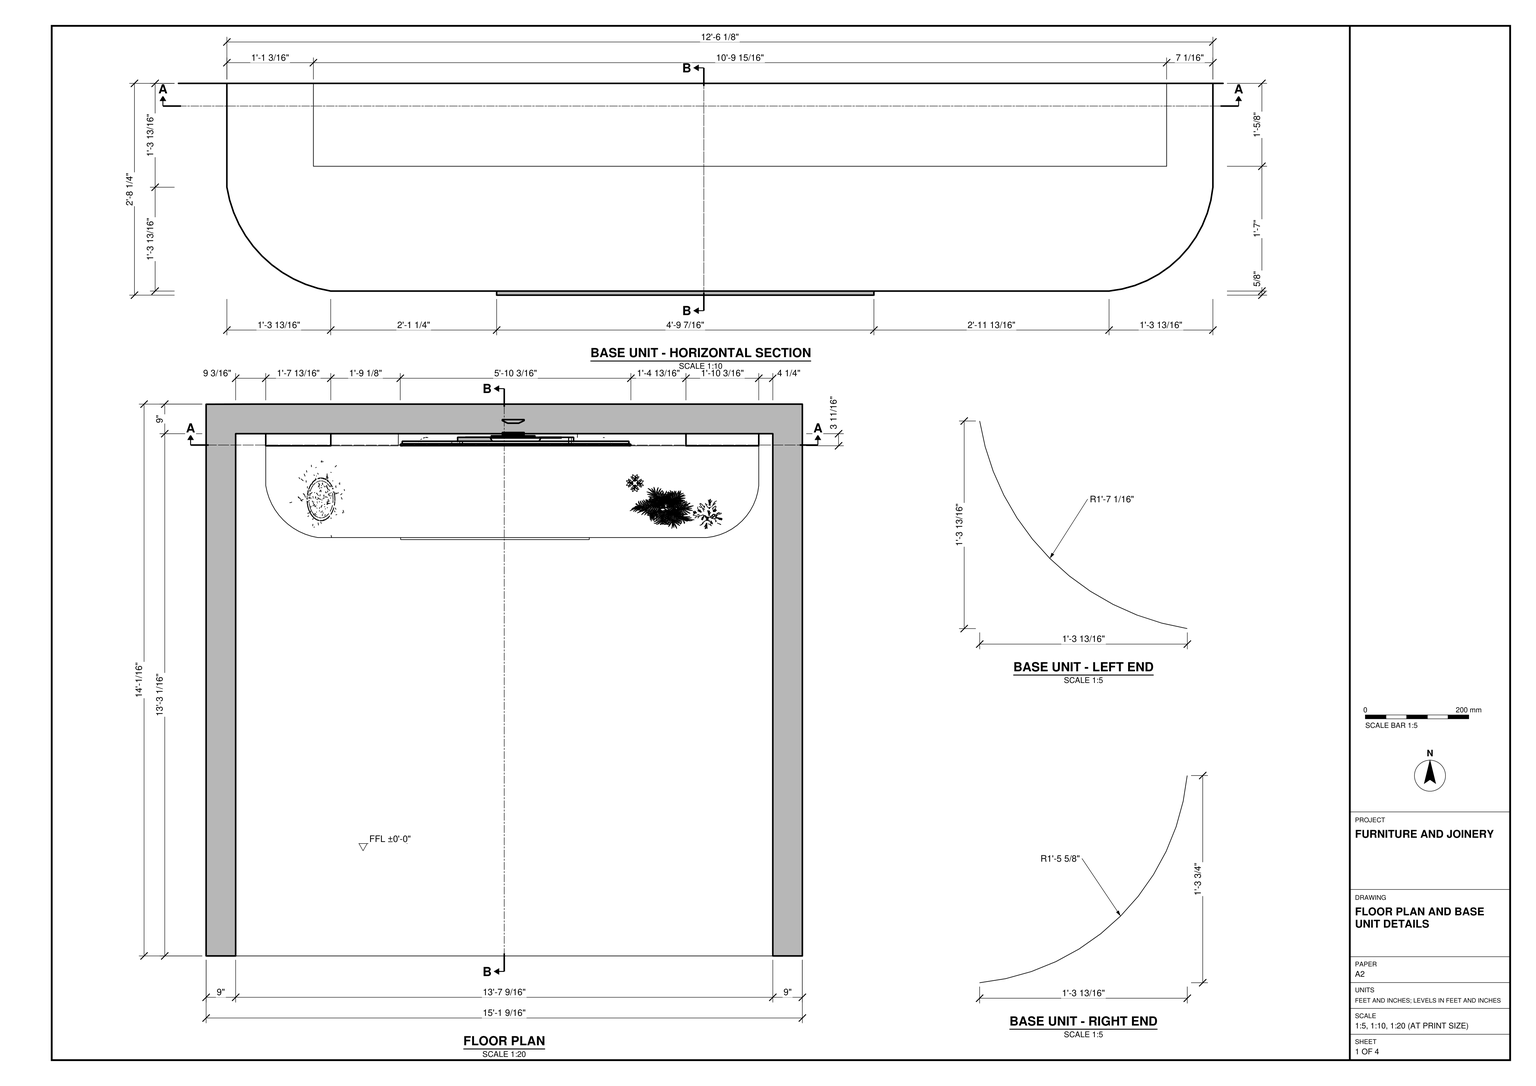
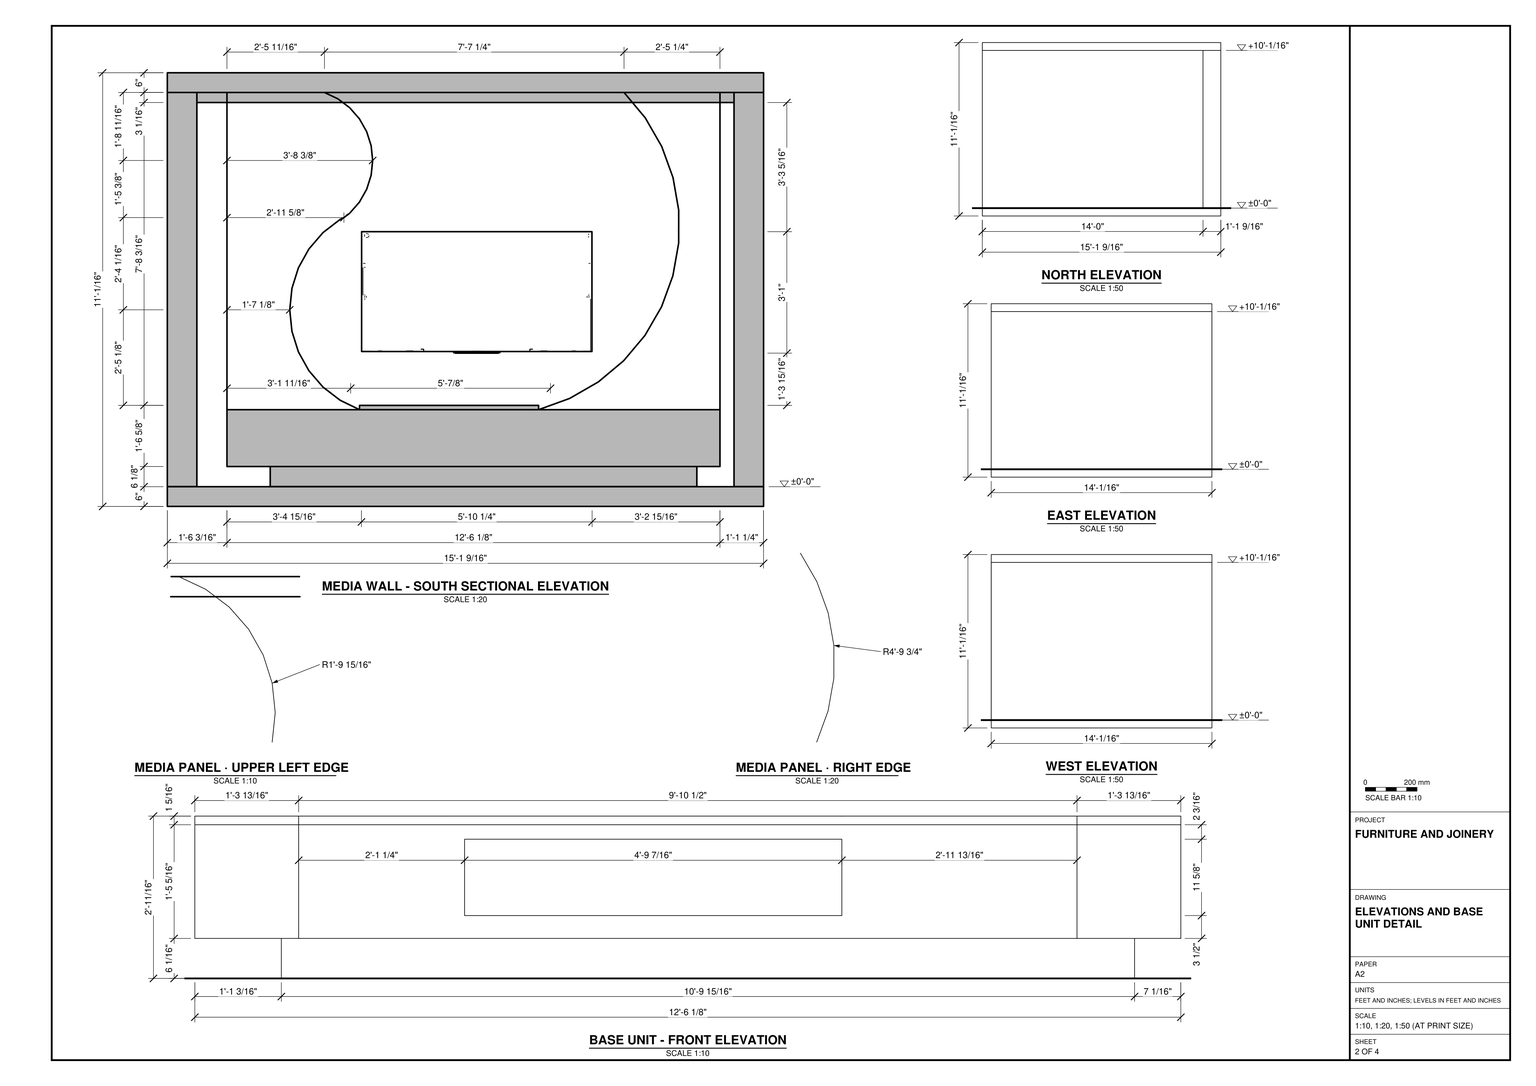
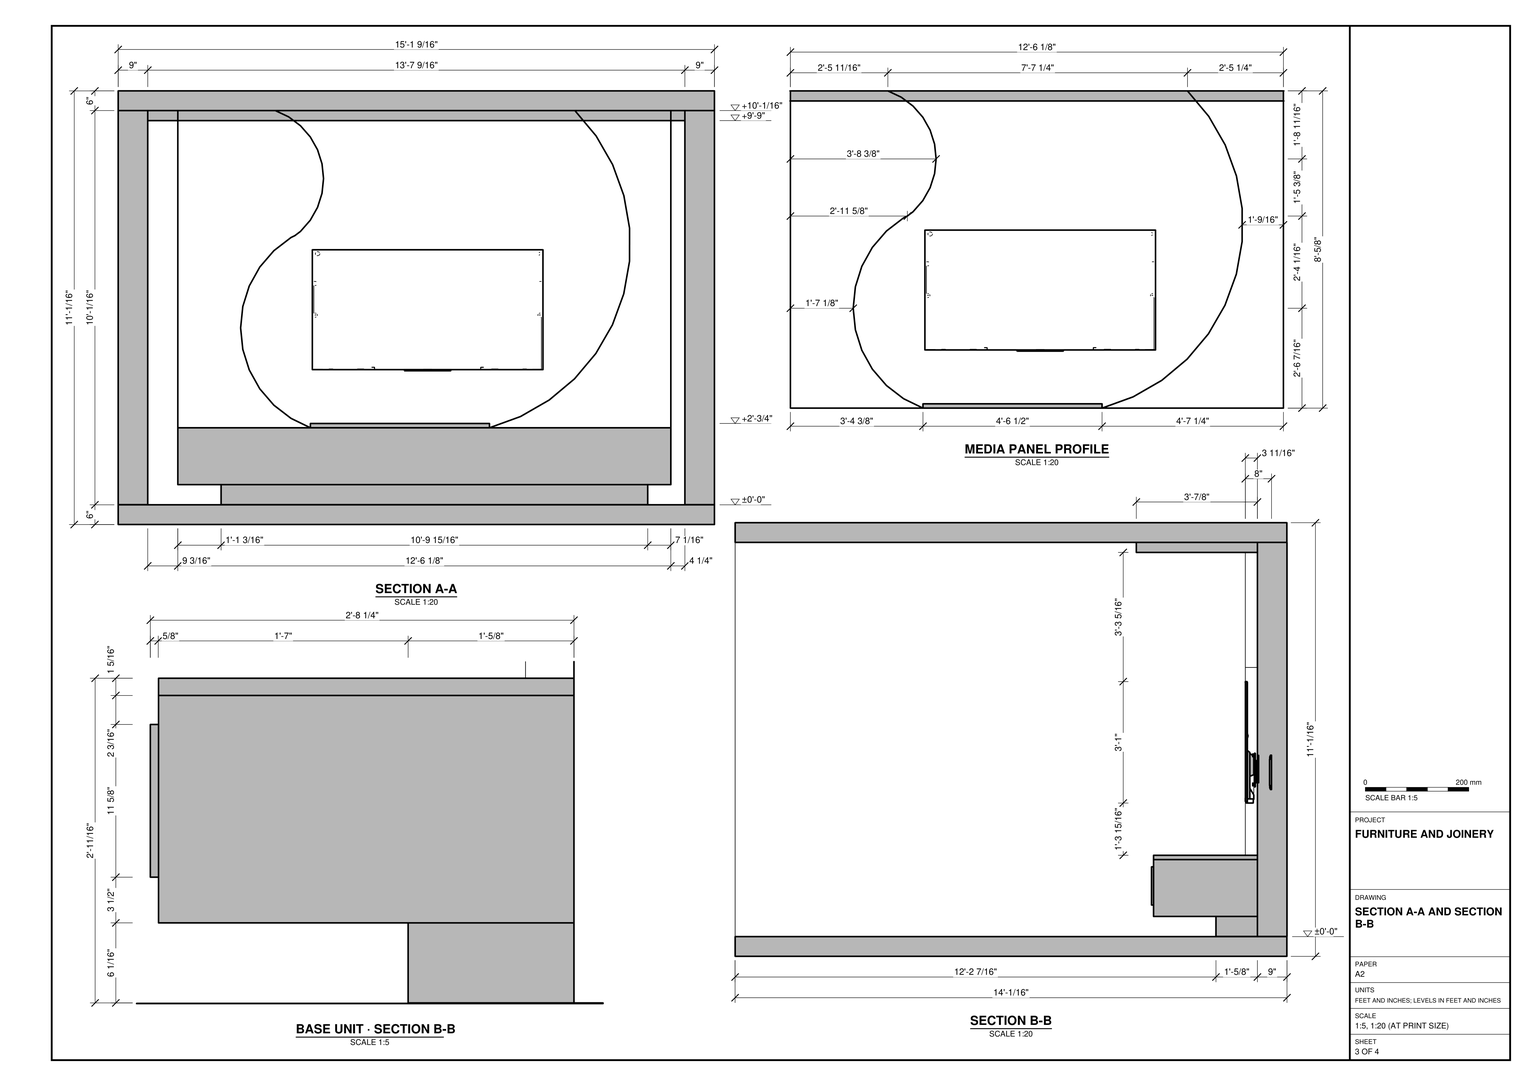
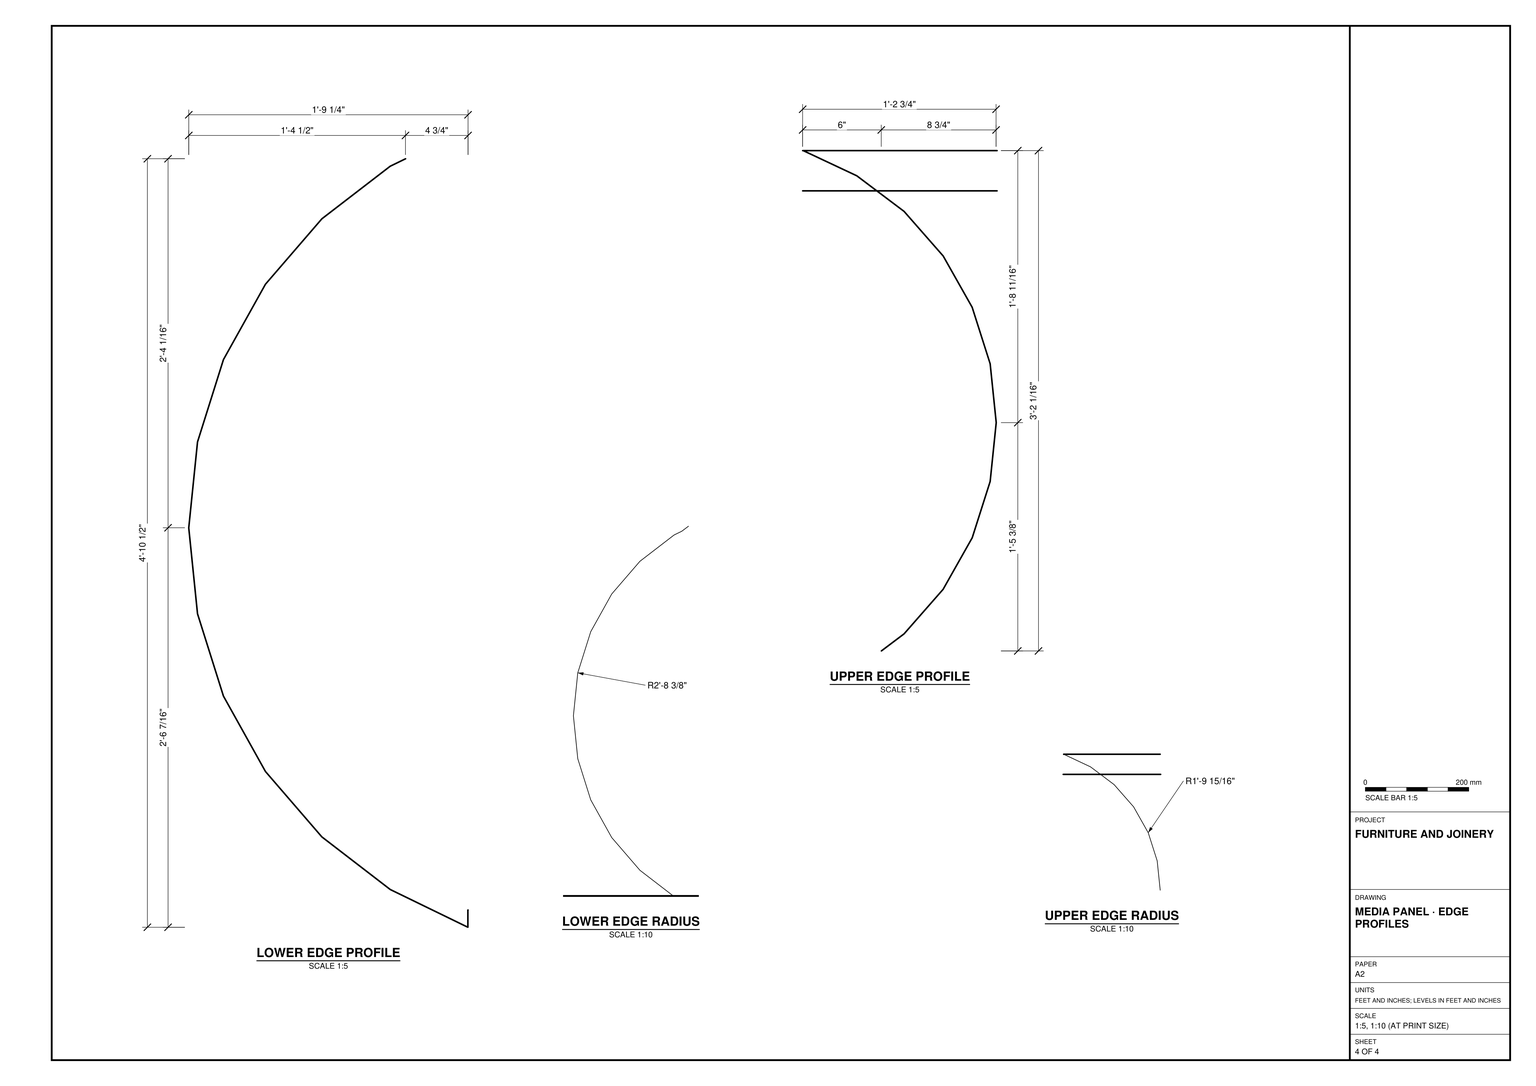
Build the media wall and its surrounding room shell in SketchUp using task_files/diagram_01.pdf. Work in feet and inches. The overall model is 15'-1 9/16" wide, 14'-1/16" deep and 11'-1/16" high, with the finished floor at ±0'-0". Form the floor slab, back wall, side walls and overhead slab, leaving the front open as shown. Use the 9" wall thickness and the slab thicknesses shown in section.

Place the base unit against the back wall, preserving the unequal clearances at its ends. Use the horizontal section and end details to shape the rounded front corners. Include the top, the projecting rectangular front panel and the recessed plinth. Above the unit, follow the media panel profile: the left edge reverses curvature, while the right edge sweeps out in a broad bow. Position the screen in front of the panel and model the shallow overhead projection shown in section. Decor and loose items, including the objects on the base unit, may be any suitable library components.

Keep the shell elements and each furniture or joinery piece in separate groups or components, and use components for repeated parts. Save one SketchUp model as output_files/media_wall_and_its_curved_base_unit.skp.

# SketchUp Ruby script. Lengths in inches.
U = 1.inch
M = Sketchup.active_model
def pt(a) = Geom::Point3d.new(a.map { |v| v * U })
def face(e, loops, mat)
  f = e.add_face(loops[0].map { |a| pt(a) })
  loops[1..].each { |l| e.add_face(l.map { |a| pt(a) }).erase! }
  f.material = f.back_material = mat if mat
  f
end
# faces: each face lists its corners as indices into pts; further lists are holes
def faces(e, pts, list, mat = nil) = list.each { |f| face(e, (f[0].is_a?(Array) ? f : [f]).map { |l| l.map { |i| pts[i] } }, mat) }
# xy, xz, yz: faces in a plane at the given z, y or x. An outline is a flat list of corners, or four numbers for a rectangle; further outlines are holes
def ring(l) = l.size == 4 ? [[l[0], l[1]], [l[2], l[1]], [l[2], l[3]], [l[0], l[3]]] : l.each_slice(2).to_a
def flat(e, list, mat, &to3) = list.each { |f| face(e, (f[0].is_a?(Array) ? f : [f]).map { |l| ring(l).map { |u, v| to3.(u, v) } }, mat) }
def xy(e, z, list, mat = nil) = flat(e, list, mat) { |x, y| [x, y, z] }
def xz(e, y, list, mat = nil) = flat(e, list, mat) { |x, z| [x, y, z] }
def yz(e, x, list, mat = nil) = flat(e, list, mat) { |y, z| [x, y, z] }
def lines(e, pts, list) = list.each { |a, b| e.add_line(pt(pts[a]), pt(pts[b])) }
# prism: a flat outline (further loops are holes) pulled along v
def prism(e, loops, v, mat = nil)
  f = face(e, loops, mat); d = Geom::Vector3d.new(v.map { |x| x * U })
  f.pushpull(f.normal.samedirection?(d) ? d.length : -d.length)
end
def box(e, o, s, mat = nil) = prism(e, [[o, [o[0] + s[0], o[1], o[2]], [o[0] + s[0], o[1] + s[1], o[2]], [o[0], o[1] + s[1], o[2]]]], [0, 0, s[2]], mat)
def at(x, y, z, deg = 0) = Geom::Transformation.translation(pt([x, y, z])) * Geom::Transformation.rotation(ORIGIN, Z_AXIS, deg.degrees)
def axes(o, x, y, z) = Geom::Transformation.new([*x, 0, *y, 0, *z, 0, *pt(o).to_a, 1])
def part(name) = M.definitions.add(name)
# library, detail: a bought-in or finely detailed component or shape, given as its bounding box
def library(name, o, s) = part(name).tap { |d| box(d.entities, o, s) }
def detail(e, o, s) = box(e.add_group.entities, o, s)
def put(e, d, t, mat = nil) = e.add_instance(d, t).tap { |i| i.material = mat if mat }
def group(e, t, mat = nil) = e.add_group.tap { |g| g.transformation = t; g.material = mat if mat }.entities
root = M.entities
M.materials.add("[Color E01]").color = [255, 255, 204]
M.materials.add("[Color M00]").color = [255, 255, 255]
M.materials.add("[Color M01]").color = [226, 226, 226]
M.materials.add("[Color M09]").color = [0, 0, 0]
M.materials.add("[Concrete Tile]").color = [203, 190, 164]
M.materials.add("[Wood Bamboo]").color = [177, 105, 43]
M.materials.add("[Wood Cherry Original]").color = [152, 86, 42]
M.materials.add("[Wood Floor Light]").color = [204, 176, 127]
c1 = library("TV WALL",[-92.5,485.99,-76.16],[49.35,7.98,28.83])
c2 = library("Vase with Flower",[-2.59,-2.59,0],[5.18,5.18,11.38])
c3 = library("2",[0,0,0],[67.42,65.5,81.95])
c4 = library("Florero",[0,-9.1,0],[22.375,11.9,13.13])
c5 = library("plant_obj1",[-93.07,-95.67,5.47],[176.43,176.66,288.74])
c6 = library("plant_obj_",[-201.12,-147.71,385.93],[345.11,315.22,326.4])
c7 = part("skpF9CrS7")
put(c7.entities,c5,at(0,0,0))
put(c7.entities,c6,at(0,-16.16,-131.76))
c8 = part("flower")
put(c8.entities,c7,at(0,0,0))
c9 = library("Omni Light\#2",[-12,-12,-12],[24,24,24])
c10 = library("Omni Light\#4",[-12,-12,-12],[24,24,24])
c11 = library("Omni Light\#5",[-12,-12,-12],[24,24,24])
c12 = library("Spot Light",[-5.1,-5.1,-11.05],[10.2,10.2,11.05])
c13 = library("Spot Light\#1",[-5.1,-5.1,-11.05],[10.2,10.2,11.05])
c14 = library("Spot Light\#3",[-5.1,-5.1,-11.05],[10.2,10.2,11.05])
c15 = library("Spot Light\#2",[-5.1,-5.1,-11.05],[10.2,10.2,11.05])
p = [[18.16,159.03,23.4],[18.16,159.03,120],[168.29,159.03,23.4],[168.29,159.03,120]]
lines(root,p,[[0,1],[2,3]])
put(root,c1,axes([190.74,-330.64,138.3125],[1.42298,0,0],[0,1,0],[0,0,1.2826]))
put(root,c2,at(130.57,143.97,24.72))
put(root,c3,axes([126.91,127.02,24.97],[0.35225,0,0],[0,0.28105,0],[0,0,0.1938]))
put(root,c4,at(136.62,137.66,26.61))
put(root,c8,axes([35.21,139.58,24.52],[0.04846,0,0],[0,0.07426,0],[0,0,0.03681]))
put(root,c9,at(149.79,134.97,110.5))
put(root,c10,at(28.01,135.16,111.75))
put(root,c11,at(90.48,123.5625,110.71))
put(root,c12,at(50.06,137.68,116.93))
put(root,c13,at(92.53,138.83,116.93))
put(root,c14,at(142.38,123.5625,110.7))
put(root,c15,at(129.35,153.59,118.27))
g1 = group(root,at(0,0,0),"[Color M01]")
xy(g1,0,[[0,0,0,168,13.5625,168.03,181.5625,168.03,181.5625,0,172.5625,0,172.5625,159.03,9,159.03,9,0]])
xy(g1,120,[[0,0,9,0,9,159.03,172.5625,159.03,172.5625,0,181.5625,0,181.5625,168.03,13.5625,168.03,0,168]])
xz(g1,0,[[0,0,9,120],[172.5625,0,181.5625,120]],"[Color M01]")
xz(g1,159.03,[[9,0,172.5625,120]],"[Color M01]")
xz(g1,168.03,[[13.5625,0,181.5625,120]])
yz(g1,0,[[0,0,168,120]])
yz(g1,9,[[0,0,159.03,120]])
yz(g1,172.5625,[[0,0,159.03,120]],"[Color M01]")
yz(g1,181.5625,[[0,0,168,120],[168,0,168.03,120]])
p = [[13.5625,168.03,0],[0,168,0],[0,168,120],[13.5625,168.03,120],[181.5625,168,0],[172.5625,168,0],
  [9,168,0]]
faces(g1,p,[[0,1,2,3]])
lines(g1,p,[[4,5],[6,1]])
g2 = group(root,at(0,0,121.125),"[Color M01]")
xy(g2,-127.18,[[0,0,181.5625,168]])
xy(g2,-121.18,[[0,0,181.5625,168]],"[Concrete Tile]")
xy(g2,-1.125,[[0,0,181.5625,168]])
xy(g2,4.875,[[0,0,181.5625,168]],"[Color M00]")
xz(g2,0,[[0,-127.18,181.5625,-121.18],[0,-1.125,181.5625,4.875]])
xz(g2,168,[[0,-127.18,181.5625,-121.18],[0,-1.125,181.5625,4.875]])
yz(g2,0,[[0,-127.18,168,-121.18],[0,-1.125,168,4.875]])
yz(g2,181.5625,[[0,-127.18,168,-121.18],[0,-1.125,168,4.875]])
g3 = group(root,at(18.16,159.03,6.09))
xy(g3,0,[[15.8125,-31.625,13.87,-31.21,11.97,-30.59,10.16,-29.78,8.43,-28.78,6.82,-27.61,5.34,-26.28,4.01,-24.8,2.84,-23.19,1.84,-21.47,1.03,-19.65,0.42,-17.76,0,-15.8125,0,0,150.125,0,150.125,-15.8125,149.8125,-17.81,149.27,-19.75,148.52,-21.62,147.55,-23.39,146.39,-25.04,145.05,-26.55,143.54,-27.89,141.89,-29.05,140.12,-30.02,138.25,-30.77,136.31,-31.3125,134.3125,-31.625]])
xy(g3,17.3125,[[0,-3.6875,40.37,0],[94.9,-3.6875,150.125,0]])
xy(g3,17.3125,[[15.8125,-31.625,13.87,-31.21,11.97,-30.59,10.16,-29.78,8.43,-28.78,6.82,-27.61,5.34,-26.28,4.01,-24.8,2.84,-23.19,1.84,-21.47,1.03,-19.65,0.42,-17.76,0,-15.8125,0,-3.6875,40.37,-3.6875,40.37,0,94.9,0,94.9,-3.6875,150.125,-3.6875,150.125,-15.8125,149.8125,-17.81,149.27,-19.75,148.52,-21.62,147.55,-23.39,146.39,-25.04,145.05,-26.55,143.54,-27.89,141.89,-29.05,140.12,-30.02,138.25,-30.77,136.31,-31.3125,134.3125,-31.625]],"[Color E01]")
xy(g3,18.625,[[15.8125,-31.625,134.3125,-31.625,136.31,-31.3125,138.25,-30.77,140.12,-30.02,141.89,-29.05,143.54,-27.89,145.05,-26.55,146.39,-25.04,147.55,-23.39,148.52,-21.62,149.27,-19.75,149.8125,-17.81,150.125,-15.8125,150.125,-3.6875,94.9,-3.6875,94.9,0,40.37,0,40.37,-3.6875,0,-3.6875,0,-15.8125,0.42,-17.76,1.03,-19.65,1.84,-21.47,2.84,-23.19,4.01,-24.8,5.34,-26.28,6.82,-27.61,8.43,-28.78,10.16,-29.78,11.97,-30.59,13.87,-31.21]],"[Wood Floor Light]")
xy(g3,113.91,[[0,-3.6875,29.68,0],[120.91,-3.6875,150.125,0]])
xz(g3,-31.625,[[15.8125,0,134.3125,17.3125]],"[Wood Cherry Original]")
xz(g3,-31.625,[[15.8125,17.3125,134.3125,18.625]],"[Wood Floor Light]")
xz(g3,-3.6875,[[40.37,17.3125,37.67,18.625,40.37,18.625],[94.9,17.3125,94.9,18.625,98.51,18.625]],"[Color E01]")
xz(g3,-3.6875,[[0,17.3125,40.37,17.3125,37.67,18.625,0,18.625],[94.9,17.3125,150.125,17.3125,150.125,18.625,98.51,18.625],[0,18.625,37.67,18.625,34.46,20.1875,29.25,24.19,24.95,29.17,21.76,34.91,19.78,41.18,19.12,47.72,19.78,54.26,21.76,60.53,24.95,66.27,29.25,71.24,32.75,73.94,34.46,75.25,35.62,75.82,37.35,77.12,40.32,80.51,40.37,80.59,42.54,84.43,43.9,88.72,44.37,93.2,43.9,97.68,42.54,101.97,40.37,105.82,40.32,105.9,37.35,109.28,33.76,111.99,29.68,113.91,0,113.91],[98.51,18.625,150.125,18.625,150.125,113.91,120.91,113.91,127.37,106.1875,132.39,97.46,135.82,88,137.56,78.08,137.54,68.01,135.78,58.1,132.33,48.65,127.28,39.93,120.8,32.23,113.08,25.77,104.36,20.74]],"[Wood Cherry Original]")
xz(g3,0,[[0,0,150.125,17.3125],[0,17.3125,0,113.91,29.68,113.91,33.76,111.99,37.35,109.28,40.32,105.9,40.37,105.82,42.54,101.97,43.9,97.68,44.37,93.2,43.9,88.72,42.54,84.43,40.37,80.59,40.32,80.51,37.35,77.12,35.62,75.82,34.46,75.25,32.75,73.94,29.25,71.24,24.95,66.27,21.76,60.53,19.78,54.26,19.12,47.72,19.78,41.18,21.76,34.91,24.95,29.17,29.25,24.19,34.46,20.1875,40.37,17.3125],[94.9,17.3125,104.36,20.74,113.08,25.77,120.8,32.23,127.28,39.93,132.33,48.65,135.78,58.1,137.54,68.01,137.56,78.08,135.82,88,132.39,97.46,127.37,106.1875,120.91,113.91,150.125,113.91,150.125,17.3125]])
xz(g3,0,[[40.37,17.3125,94.9,18.625]],"[Color E01]")
yz(g3,0,[[-15.8125,0,0,17.3125],[-3.6875,17.3125,0,113.91]])
yz(g3,0,[[-15.8125,17.3125,-3.6875,18.625]],"[Color E01]")
yz(g3,40.37,[[-3.6875,17.3125,0,18.625]],"[Color E01]")
yz(g3,94.9,[[-3.6875,17.3125,0,18.625]],"[Color E01]")
yz(g3,150.125,[[-15.8125,0,0,17.3125],[-3.6875,17.3125,0,113.91]])
yz(g3,150.125,[[-15.8125,17.3125,-3.6875,18.625]],"[Color E01]")
p = [[15.8125,-31.625,17.3125],[13.87,-31.21,17.3125],[13.87,-31.21,0],[15.8125,-31.625,0],[136.31,-31.3125,17.3125],[134.3125,-31.625,17.3125],
  [134.3125,-31.625,0],[136.31,-31.3125,0],[138.25,-30.77,17.3125],[138.25,-30.77,0],[11.97,-30.59,17.3125],[11.97,-30.59,0],
  [140.12,-30.02,17.3125],[140.12,-30.02,0],[10.16,-29.78,17.3125],[10.16,-29.78,0],[141.89,-29.05,17.3125],[141.89,-29.05,0],
  [8.43,-28.78,17.3125],[8.43,-28.78,0],[143.54,-27.89,17.3125],[143.54,-27.89,0],[6.82,-27.61,17.3125],[6.82,-27.61,0],
  [145.05,-26.55,17.3125],[145.05,-26.55,0],[5.34,-26.28,17.3125],[5.34,-26.28,0],[146.39,-25.04,17.3125],[146.39,-25.04,0],
  [4.01,-24.8,17.3125],[4.01,-24.8,0],[147.55,-23.39,17.3125],[147.55,-23.39,0],[2.84,-23.19,17.3125],[2.84,-23.19,0],
  [148.52,-21.62,17.3125],[148.52,-21.62,0],[1.84,-21.47,17.3125],[1.84,-21.47,0],[149.27,-19.75,17.3125],[149.27,-19.75,0],
  [1.03,-19.65,17.3125],[1.03,-19.65,0],[149.8125,-17.81,17.3125],[149.8125,-17.81,0],[0.42,-17.76,17.3125],[0.42,-17.76,0],
  [0,-15.8125,17.3125],[0,-15.8125,0],[150.125,-15.8125,17.3125],[150.125,-15.8125,0],[15.8125,-31.625,18.625],[13.87,-31.21,18.625],
  [136.31,-31.3125,18.625],[134.3125,-31.625,18.625],[138.25,-30.77,18.625],[11.97,-30.59,18.625],[140.12,-30.02,18.625],[10.16,-29.78,18.625],
  [141.89,-29.05,18.625],[8.43,-28.78,18.625],[143.54,-27.89,18.625],[6.82,-27.61,18.625],[145.05,-26.55,18.625],[5.34,-26.28,18.625],
  [146.39,-25.04,18.625],[4.01,-24.8,18.625],[147.55,-23.39,18.625],[2.84,-23.19,18.625],[148.52,-21.62,18.625],[1.84,-21.47,18.625],
  [149.27,-19.75,18.625],[1.03,-19.65,18.625],[149.8125,-17.81,18.625],[0.42,-17.76,18.625],[0,-15.8125,18.625],[150.125,-15.8125,18.625],
  [40.37,0,17.3125],[34.46,0,20.1875],[34.46,-3.6875,20.1875],[37.67,-3.6875,18.625],[40.37,-3.6875,17.3125],[104.36,0,20.74],
  [94.9,0,17.3125],[94.9,-3.6875,17.3125],[98.51,-3.6875,18.625],[104.36,-3.6875,20.74],[29.25,0,24.19],[29.25,-3.6875,24.19],
  [113.08,0,25.77],[113.08,-3.6875,25.77],[24.95,0,29.17],[24.95,-3.6875,29.17],[120.8,0,32.23],[120.8,-3.6875,32.23],
  [21.76,0,34.91],[21.76,-3.6875,34.91],[127.28,0,39.93],[127.28,-3.6875,39.93],[19.78,0,41.18],[19.78,-3.6875,41.18],
  [132.33,0,48.65],[132.33,-3.6875,48.65],[19.12,0,47.72],[19.12,-3.6875,47.72],[19.78,0,54.26],[19.78,-3.6875,54.26],
  [135.78,0,58.1],[135.78,-3.6875,58.1],[21.76,0,60.53],[21.76,-3.6875,60.53],[137.54,0,68.01],[137.54,-3.6875,68.01],
  [24.95,0,66.27],[24.95,-3.6875,66.27],[29.25,0,71.24],[29.25,-3.6875,71.24],[137.56,0,78.08],[137.56,-3.6875,78.08],
  [32.75,0,73.94],[32.75,-3.6875,73.94],[34.46,0,75.25],[34.46,-3.6875,75.25],[35.62,0,75.82],[35.62,-3.6875,75.82],
  [37.35,0,77.12],[37.35,-3.6875,77.12],[40.32,0,80.51],[40.32,-3.6875,80.51],[135.82,0,88],[135.82,-3.6875,88],
  [40.37,0,80.59],[40.37,-3.6875,80.59],[42.54,0,84.43],[42.54,-3.6875,84.43],[43.9,0,88.72],[43.9,-3.6875,88.72],
  [132.39,0,97.46],[132.39,-3.6875,97.46],[44.37,0,93.2],[44.37,-3.6875,93.2],[43.9,0,97.68],[43.9,-3.6875,97.68],
  [127.37,0,106.1875],[127.37,-3.6875,106.1875],[42.54,0,101.97],[42.54,-3.6875,101.97],[40.37,0,105.82],[40.37,-3.6875,105.82],
  [40.32,0,105.9],[40.32,-3.6875,105.9],[37.35,0,109.28],[37.35,-3.6875,109.28],[120.91,0,113.91],[120.91,-3.6875,113.91],
  [33.76,0,111.99],[33.76,-3.6875,111.99],[29.68,0,113.91],[29.68,-3.6875,113.91]]
faces(g3,p,[[0,1,2,3],[4,5,6,7],[8,4,7,9],[1,10,11,2],[12,8,9,13],[10,14,15,11],[16,12,13,17],[14,18,19,15],
  [20,16,17,21],[18,22,23,19],[24,20,21,25],[22,26,27,23],[28,24,25,29],[26,30,31,27],[32,28,29,33],[30,34,35,31],
  [36,32,33,37],[34,38,39,35],[40,36,37,41],[38,42,43,39],[44,40,41,45],[42,46,47,43],[46,48,49,47],[50,44,45,51]],"[Wood Cherry Original]")
faces(g3,p,[[1,0,52,53],[5,4,54,55],[4,8,56,54],[10,1,53,57],[8,12,58,56],[14,10,57,59],[12,16,60,58],[18,14,59,61],
  [16,20,62,60],[22,18,61,63],[20,24,64,62],[26,22,63,65],[24,28,66,64],[30,26,65,67],[28,32,68,66],[34,30,67,69],
  [32,36,70,68],[38,34,69,71],[36,40,72,70],[42,38,71,73],[40,44,74,72],[46,42,73,75],[48,46,75,76],[44,50,77,74]],"[Wood Floor Light]")
faces(g3,p,[[78,79,80,81,82],[83,84,85,86,87],[79,88,89,80],[90,83,87,91],[88,92,93,89],[94,90,91,95],[92,96,97,93],[98,94,95,99],
  [96,100,101,97],[102,98,99,103],[100,104,105,101],[104,106,107,105],[108,102,103,109],[106,110,111,107],[112,108,109,113],[110,114,115,111],
  [114,116,117,115],[118,112,113,119],[116,120,121,117],[120,122,123,121],[122,124,125,123],[124,126,127,125],[126,128,129,127],[130,118,119,131],
  [128,132,133,129],[132,134,135,133],[134,136,137,135],[138,130,131,139],[136,140,141,137],[140,142,143,141],[144,138,139,145],[142,146,147,143],
  [146,148,149,147],[148,150,151,149],[150,152,153,151],[154,144,145,155],[152,156,157,153],[156,158,159,157]])
g4 = group(root,at(31.34,159.03,0))
box(g4,[0,-12.625,0],[129.91,12.625,6.09],"[Wood Bamboo]")
g5 = group(root,at(59.24,127.41,9.57))
xy(g5,0,[[0,-0.625,57.4375,0]])
xy(g5,11.625,[[0,-0.625,57.4375,0]])
xz(g5,-0.625,[[0,0,57.4375,11.625]],"[Color M09]")
xz(g5,0,[[0,0,57.4375,11.625]])
yz(g5,0,[[-0.625,0,0,11.625]])
yz(g5,57.4375,[[-0.625,0,0,11.625]])
g6 = group(root,at(9,122.16,120))
prism(g6,[[[0,36.88,-3.0625],[9.16,36.88,-3.0625],[159.29,36.88,-3.0625],[163.5625,36.88,-3.0625],[163.5625,0,-3.0625],[0,0,-3.0625]]],[0,0,3.0625])
